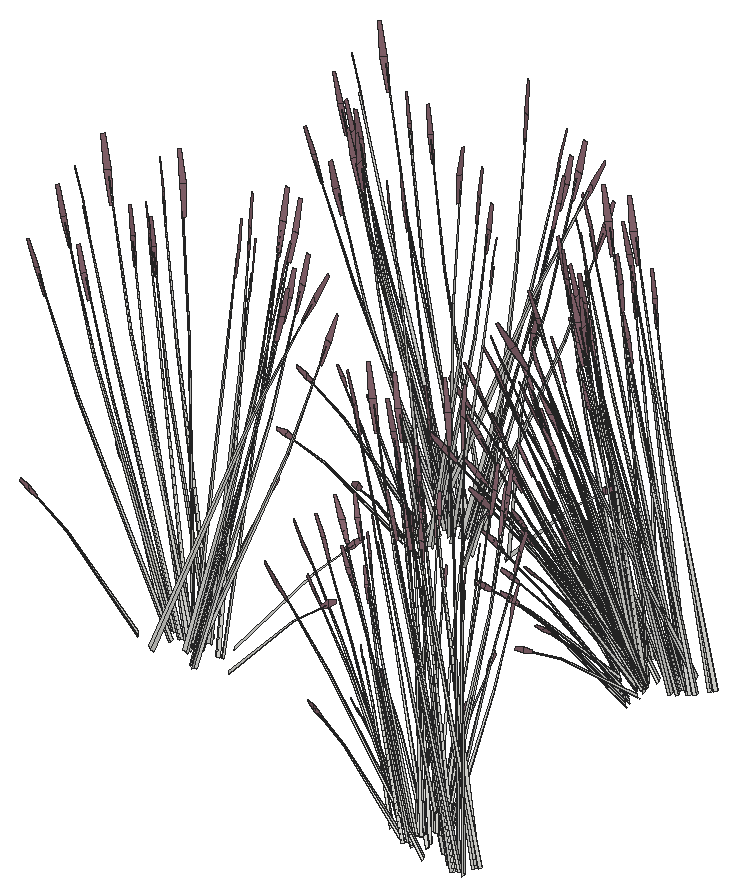
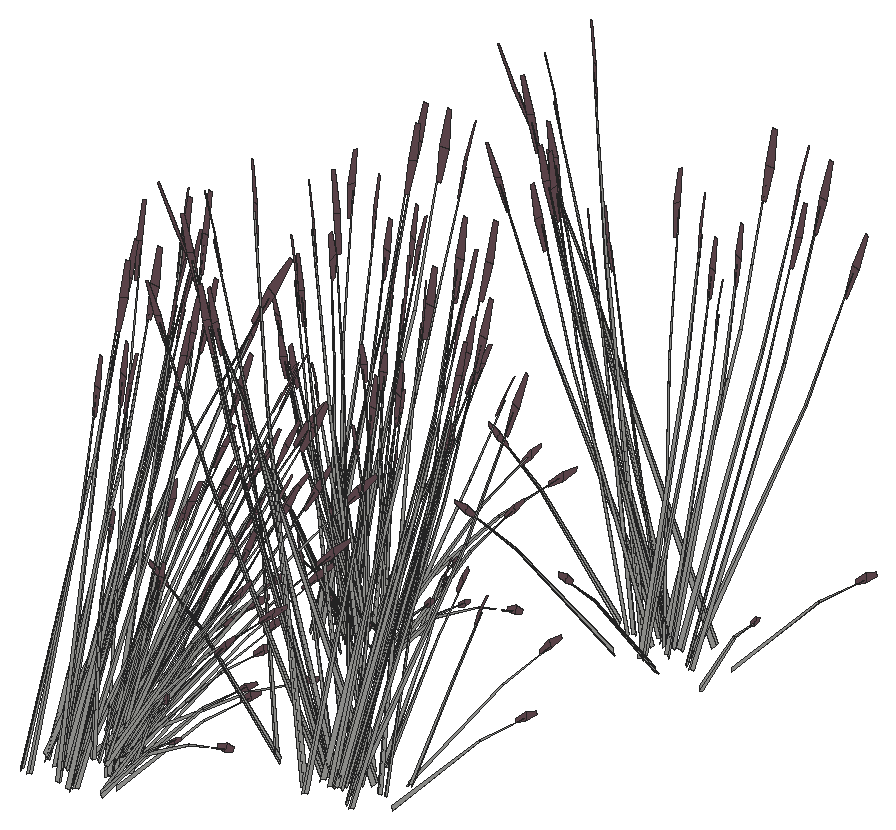
# SketchUp Ruby script. Lengths in inches.
U = 1.inch
M = Sketchup.active_model
def pt(a) = Geom::Point3d.new(a.map { |v| v * U })
def face(e, loops, mat)
  f = e.add_face(loops[0].map { |a| pt(a) })
  loops[1..].each { |l| e.add_face(l.map { |a| pt(a) }).erase! }
  f.material = f.back_material = mat if mat
  f
end
# faces: each face lists its corners as indices into pts; further lists are holes
def faces(e, pts, list, mat = nil) = list.each { |f| face(e, (f[0].is_a?(Array) ? f : [f]).map { |l| l.map { |i| pts[i] } }, mat) }
# xy, xz, yz: faces in a plane at the given z, y or x. An outline is a flat list of corners, or four numbers for a rectangle; further outlines are holes
def ring(l) = l.size == 4 ? [[l[0], l[1]], [l[2], l[1]], [l[2], l[3]], [l[0], l[3]]] : l.each_slice(2).to_a
def flat(e, list, mat, &to3) = list.each { |f| face(e, (f[0].is_a?(Array) ? f : [f]).map { |l| ring(l).map { |u, v| to3.(u, v) } }, mat) }
def xy(e, z, list, mat = nil) = flat(e, list, mat) { |x, y| [x, y, z] }
def xz(e, y, list, mat = nil) = flat(e, list, mat) { |x, z| [x, y, z] }
def yz(e, x, list, mat = nil) = flat(e, list, mat) { |y, z| [x, y, z] }
def lines(e, pts, list) = list.each { |a, b| e.add_line(pt(pts[a]), pt(pts[b])) }
# prism: a flat outline (further loops are holes) pulled along v
def prism(e, loops, v, mat = nil)
  f = face(e, loops, mat); d = Geom::Vector3d.new(v.map { |x| x * U })
  f.pushpull(f.normal.samedirection?(d) ? d.length : -d.length)
end
def box(e, o, s, mat = nil) = prism(e, [[o, [o[0] + s[0], o[1], o[2]], [o[0] + s[0], o[1] + s[1], o[2]], [o[0], o[1] + s[1], o[2]]]], [0, 0, s[2]], mat)
def at(x, y, z, deg = 0) = Geom::Transformation.translation(pt([x, y, z])) * Geom::Transformation.rotation(ORIGIN, Z_AXIS, deg.degrees)
def axes(o, x, y, z) = Geom::Transformation.new([*x, 0, *y, 0, *z, 0, *pt(o).to_a, 1])
def part(name) = M.definitions.add(name)
# library, detail: a bought-in or finely detailed component or shape, given as its bounding box
def library(name, o, s) = part(name).tap { |d| box(d.entities, o, s) }
def detail(e, o, s) = box(e.add_group.entities, o, s)
def put(e, d, t, mat = nil) = e.add_instance(d, t).tap { |i| i.material = mat if mat }
def group(e, t, mat = nil) = e.add_group.tap { |g| g.transformation = t; g.material = mat if mat }.entities
root = M.entities
M.materials.add("LightPink_Translucent").color = [144, 107, 117]
c1 = part("blade")
p = [[2.15,0.21,22],[0,0.17,0],[0.09,0.45,0],[2.18,0.31,22],[2.29,0.31,22],[0.38,0.45,0],
  [2.48,0.24,33],[2.49,0.24,33],[2.48,0.22,33]]
faces(c1.entities,p,[[0,1,2,3],[4,5,2,3],[6,3,4,7],[8,0,3,6]])
c2 = part("seeds")
p = [[0.3,-0.1,1.38],[-0.01,-0.03,1.59],[-0.01,-0.03,0.03],[0.14,-0.07,-0.07],[0.29,-0.03,3],[0.15,0.01,3.11]]
faces(c2.entities,p,[[0,1,2,3],[1,0,4,5]],"LightPink_Translucent")
c3 = part("blade with seeds")
put(c3.entities,c1,at(0,0,0))
put(c3.entities,c2,axes([2.4,0.25,30.99],[1.5799,-0.05474,1.17369],[-0.12525,1.92788,0.29478],[-0.07173,-0.02425,1.56792]))
put(root,c3,axes([28.59,392.67,43.49],[0.03108,0.16322,1.76342],[-0.62654,0.85237,-0.26939],[-0.44504,-0.04296,0.30037]))
put(root,c3,axes([28.26,397.24,43.49],[0.16438,0.10347,1.76342],[0.27873,0.95868,-0.26939],[-0.36432,0.20444,0.30037]))
put(root,c3,axes([32.69,394.15,44.06],[-1.27479,-0.1698,-0.62353],[0.26901,-1.04736,-0.16365],[-0.38043,-0.12691,1.37633]))
put(root,c3,axes([31.02,396.14,44.02],[-1.14694,-0.51783,-0.49651],[0.68554,-0.92854,0],[-0.26122,-0.11794,1.57504]))
put(root,c3,axes([34.14,394.31,44.67],[-1.23732,0.68758,-0.29095],[-0.8228,-0.97154,-0.50002],[-0.30528,-0.09867,1.59708]))
put(root,c3,axes([31.34,395.75,44.03],[-0.28787,-0.90242,-0.30978],[1.14332,-0.25625,0.30978],[-0.23049,-0.10406,1.38974]))
put(root,c3,axes([34.96,395.06,44.06],[-0.82544,0.77843,-0.62353],[-1.0254,-0.70586,-0.16365],[-0.33076,0.19418,1.37633]))
put(root,c3,axes([35.53,394.62,44.46],[-1.19666,-0.83357,-0.25192],[1.00694,-0.93603,0.5513],[-0.32224,0.09751,1.68216]))
put(root,c3,axes([36.74,432.36,43.49],[0.03108,0.16322,1.76342],[-0.62654,0.85237,-0.26939],[-0.44504,-0.04296,0.30037]))
put(root,c3,axes([34.92,394.44,44.21],[-1.33077,0.06393,-0.44739],[-0.12035,-1.06125,0.21531],[-0.23824,0.10756,1.43643]))
put(root,c3,axes([36.32,397.18,44.02],[-1.14694,0.51783,-0.49651],[-0.68554,-0.92854,0],[-0.26122,0.11794,1.57504]))
put(root,c3,axes([36.05,396.77,44.03],[-1.14332,-0.25625,-0.30978],[0.28787,-0.90242,0.30978],[-0.23049,0.10406,1.38974]))
put(root,c3,axes([35.85,394.16,44.67],[0.1428,1.18174,-0.29095],[-1.48733,0.07145,-0.50002],[-0.26191,0.15741,1.59708]))
put(root,c3,axes([40.84,433.84,44.06],[-1.27479,-0.1698,-0.62353],[0.26901,-1.04736,-0.16365],[-0.38043,-0.12691,1.37633]))
put(root,c3,axes([39.17,435.83,44.02],[-1.14694,-0.51783,-0.49651],[0.68554,-0.92854,0],[-0.26122,-0.11794,1.57504]))
put(root,c3,axes([38.67,428.11,43.49],[-0.11871,0.13643,1.76342],[-1.19964,0.29415,-0.26939],[-0.2898,-0.26759,0.30037]))
put(root,c3,axes([37.92,428.64,44.13],[-0.35352,0.84566,-0.03893],[-1.08806,-0.26014,-0.17649],[-0.1652,-0.13832,0.58215]))
put(root,c3,axes([33.33,397.34,43.49],[0.19833,-0.05635,1.76342],[1.19302,0.31018,-0.26939],[0.03489,0.3496,0.30037]))
put(root,c3,axes([42.29,434,44.67],[-1.23732,0.68758,-0.29095],[-0.8228,-0.97154,-0.50002],[-0.30528,-0.09867,1.59708]))
put(root,c3,axes([39.49,435.44,44.03],[-0.28787,-0.90242,-0.30978],[1.14332,-0.25625,0.30978],[-0.23049,-0.10406,1.38974]))
put(root,c3,axes([36.4,393.69,44.21],[-0.59459,0.93321,-0.44739],[-1.23546,-0.44912,0.21531],[0,0.21512,1.43643]))
put(root,c3,axes([43.68,434.3125,44.46],[-1.19666,-0.83357,-0.25192],[1.00694,-0.93603,0.5513],[-0.32224,0.09751,1.68216]))
put(root,c3,axes([41.5,433.51,44.21],[-0.73619,-0.86927,-0.44739],[1.11511,-0.61213,0.21531],[-0.23824,-0.10756,1.43643]))
put(root,c3,axes([43.07,434.14,44.21],[-1.33077,0.06393,-0.44739],[-0.12035,-1.06125,0.21531],[-0.23824,0.10756,1.43643]))
put(root,c3,axes([41.61,434.01,44.4375],[0.32481,-1.2272,-0.23429],[1.54007,0.21392,0.51271],[-0.26911,-0.16947,1.5644]))
put(root,c3,axes([37.68,431.71,44.02],[0,-1.03566,-0.49651],[1.37109,0,0],[0,-0.23588,1.57504]))
put(root,c3,axes([39.54,394.09,44.03],[-0.85545,0.64616,-0.30978],[-0.85545,-0.64616,0.30978],[0,0.20813,1.38974]))
put(root,c3,axes([37.09,393.98,44.09],[0.44936,0.94823,-0.69212],[-1.29441,0.3415,-0.18165],[0.04967,0.32109,1.52773]))
put(root,c3,axes([44.2,436.46,44.03],[-1.14332,-0.25625,-0.30978],[0.28787,-0.90242,0.30978],[-0.23049,0.10406,1.38974]))
put(root,c3,axes([41.26,432.91,44.67],[-1.38012,-0.49416,-0.29095],[0.66454,-1.04299,-0.50002],[-0.04337,-0.25608,1.59708]))
put(root,c3,axes([36.54,392.92,44.67],[1.38012,0.49416,-0.29095],[-0.66454,1.04299,-0.50002],[0.04337,0.25608,1.59708]))
put(root,c3,axes([40.65,431.86,44.1],[-0.50328,-1.06202,-0.69835],[1.44974,-0.38248,-0.18329],[-0.05563,-0.35963,1.54149]))
put(root,c3,axes([38.27,431.74,44.03],[0.85545,-0.64616,-0.30978],[0.85545,0.64616,0.30978],[0,-0.20813,1.38974]))
put(root,c3,axes([42.13,427.56,44.13],[-0.84686,0.59414,-0.03893],[-0.77596,-0.65071,-0.17649],[-0.05463,-0.18438,0.58215]))
put(root,c3,axes([40.125,394.12,44.02],[0,1.03566,-0.49651],[-1.37109,0,0],[0,0.23588,1.57504]))
put(root,c3,axes([36.28,395.33,44.18],[1.2866,-0.3514,-0.19198],[0.45209,1.01223,0.00008],[0.14202,-0.03884,1.73897]))
put(root,c3,axes([36.3,392.32,44.21],[0.73619,0.86927,-0.44739],[-1.11511,0.61213,0.21531],[0.23824,0.10756,1.43643]))
put(root,c3,axes([42.34,426.83,43.49],[-0.20555,0.03731,1.76342],[-1.13672,-0.42002,-0.26939],[0.01907,-0.35034,0.30037]))
put(root,c3,axes([41.41,432.14,44.21],[0.59459,-0.93321,-0.44739],[1.23546,0.44912,0.21531],[0,-0.21512,1.43643]))
put(root,c3,axes([38.32,390.39,44.03],[0.28787,0.90242,-0.30978],[-1.14332,0.25625,0.30978],[0.23049,0.10406,1.38974]))
put(root,c3,axes([35.52,391.83,44.67],[1.23732,-0.68758,-0.29095],[0.8228,0.97154,-0.50002],[0.30528,0.09867,1.59708]))
put(root,c3,axes([32.39,391.22,43.59],[-1.20625,0.41464,1.28929],[-0.38394,-1.1897,0.50096],[0.74071,0.01979,1.46642]))
put(root,c3,axes([38.64,390,44.02],[1.14694,0.51783,-0.49651],[-0.68554,0.92854,0],[0.26122,0.11794,1.57504]))
put(root,c3,axes([38.58,397.37,43.49],[0.08928,-0.14952,1.76342],[1.12407,-0.44035,-0.26939],[0.34078,0.22791,0.30037]))
put(root,c3,axes([36.96,391.99,44.06],[1.27479,0.1698,-0.62353],[-0.26901,1.04736,-0.16365],[0.38043,0.12691,1.37633]))
put(root,c3,axes([41.95,431.67,44.67],[-0.1428,-1.18174,-0.29095],[1.48733,-0.07145,-0.50002],[0.26191,-0.15741,1.59708]))
put(root,c3,axes([41.76,429.06,44.03],[1.14332,0.25625,-0.30978],[-0.28787,0.90242,0.30978],[0.23049,-0.10406,1.38974]))
put(root,c3,axes([41.49,428.65,44.02],[1.14694,-0.51783,-0.49651],[0.68554,0.92854,0],[0.26122,-0.11794,1.57504]))
put(root,c3,axes([44.43,435.02,44.18],[1.2866,-0.3514,-0.19198],[0.45209,1.01223,0.00008],[0.14202,-0.03884,1.73897]))
put(root,c3,axes([44.46,432.01,44.21],[0.73619,0.86927,-0.44739],[-1.11511,0.61213,0.21531],[0.23824,0.10756,1.43643]))
put(root,c3,axes([41.82,392.83,43.49],[-0.06405,-0.15723,1.76342],[0.44421,-0.91974,-0.26939],[0.4481,-0.01323,0.30037]))
put(root,c3,axes([42.85,430.77,44.06],[0.82544,-0.77843,-0.62353],[1.0254,0.70586,-0.16365],[0.33076,-0.19418,1.37633]))
put(root,c3,axes([46.47,430.08,44.03],[0.28787,0.90242,-0.30978],[-1.14332,0.25625,0.30978],[0.23049,0.10406,1.38974]))
put(root,c3,axes([43.67,431.52,44.67],[1.23732,-0.68758,-0.29095],[0.8228,0.97154,-0.50002],[0.30528,0.09867,1.59708]))
put(root,c3,axes([40.55,430.91,43.59],[-1.20625,0.41464,1.28929],[-0.38394,-1.1897,0.50096],[0.74071,0.01979,1.46642]))
put(root,c3,axes([47.375,428.62,43.49],[-0.18342,-0.08159,1.76342],[-0.47115,-0.9115,-0.26939],[0.31784,-0.24736,0.30037]))
put(root,c3,axes([46.79,429.7,44.02],[1.14694,0.51783,-0.49651],[-0.68554,0.92854,0],[0.26122,0.11794,1.57504]))
put(root,c3,axes([45.12,431.68,44.06],[1.27479,0.1698,-0.62353],[-0.26901,1.04736,-0.16365],[0.38043,0.12691,1.37633]))
put(root,c3,axes([50.54,432.3,44.26],[-0.75977,-0.66224,-0.06488],[0.83212,-0.6068,-0.29416],[0.23578,-0.04272,0.97024]))
put(root,c3,axes([69.75,430.67,36.3],[0.50831,-0.02346,1.71376],[-0.33721,1.01661,0.13857],[-0.72439,-0.06288,0.73262]))
put(root,c3,axes([49.97,432.53,43.49],[-0.06405,-0.15723,1.76342],[0.44421,-0.91974,-0.26939],[0.4481,-0.01323,0.30037]))
put(root,c3,axes([69.96,389.98,32.11],[0.42521,-0.21906,1.71376],[0.35798,1.01226,0.13857],[-0.66754,0.22878,0.73262]))
put(root,c3,axes([69.96,432.46,36.3],[0.42521,-0.21906,1.71376],[0.35798,1.01226,0.13857],[-0.66754,0.22878,0.73262]))
put(root,c3,axes([68.64,391.7,30.83],[0.42589,0.08502,1.43002],[0.2745,0.86839,-0.30754],[-0.57851,0.16255,0.61141]))
put(root,c3,axes([68.64,434.1875,35.02],[0.42589,0.08502,1.43002],[0.2745,0.86839,-0.30754],[-0.57851,0.16255,0.61141]))
put(root,c3,axes([72.41,388.92,31.58],[0.34834,-0.14982,1.77064],[0.12012,1.04605,0.13857],[-0.75452,0.1388,0.63284]))
put(root,c3,axes([72.41,431.41,35.77],[0.34834,-0.14982,1.77064],[0.12012,1.04605,0.13857],[-0.75452,0.1388,0.63284]))
put(root,c3,axes([68.66,389.62,32.95],[-0.20012,0.13446,1.74944],[0.01702,0.98243,-0.27667],[-0.45871,0.12776,0.14031]))
put(root,c3,axes([68.66,432.11,37.14],[-0.20012,0.13446,1.74944],[0.01702,0.98243,-0.27667],[-0.45871,0.12776,0.14031]))
put(root,c3,axes([71.27,429.73,37.41],[-1.22504,-0.02494,-0.71045],[0.08228,-1.05005,0.08574],[-0.51899,-0.11081,1.00501]))
put(root,c3,axes([70.29,429.98,35.02],[0.23927,0.28834,1.43002],[-0.55135,0.78376,-0.30754],[-0.56612,-0.18733,0.61141]))
put(root,c3,axes([69.31,431.55,36.95],[-1.01846,-0.28891,-0.35414],[0.29705,-0.84289,0.4572],[-0.41005,0.07729,0.87481]))
put(root,c3,axes([70.71,429.04,36.3],[0.45521,0.17844,1.71376],[-0.94204,0.74856,0.13857],[-0.58713,-0.33769,0.73262]))
put(root,c3,axes([66.4375,390.62,32.95],[0.1564,0.02778,1.77383],[0.48382,0.91506,-0.16761],[-0.32016,0.24017,0.31391]))
put(root,c3,axes([66.4375,433.1,37.14],[0.1564,0.02778,1.77383],[0.48382,0.91506,-0.16761],[-0.32016,0.24017,0.31391]))
put(root,c3,axes([70,389.49,32.92],[-0.332,0.94205,-0.51099],[-1.13828,-0.3229,-0.3958],[-0.45829,0.08638,0.97773]))
put(root,c3,axes([70,431.98,37.11],[-0.332,0.94205,-0.51099],[-1.13828,-0.3229,-0.3958],[-0.45829,0.08638,0.97773]))
put(root,c3,axes([70.87,429.94,37.11],[-0.88986,0.68603,-0.51099],[-0.77932,-0.72471,-0.3958],[-0.45212,-0.10438,0.97773]))
put(root,c3,axes([69.43,431.92,33.92],[0.03108,0.16322,1.76342],[-0.62654,0.85237,-0.26939],[-0.44504,-0.04296,0.30037]))
put(root,c3,axes([69.61,428.02,37.14],[0.09085,0.10335,1.77383],[-0.43798,0.92907,-0.16761],[-0.44357,0.00672,0.31391]))
put(root,c3,axes([67.75,393.52,31],[0.51072,-0.46938,1.1486],[0.20153,0.74307,0.84392],[-0.36908,0.13305,0.25299]))
put(root,c3,axes([67.75,436.01,35.19],[0.51072,-0.46938,1.1486],[0.20153,0.74307,0.84392],[-0.36908,0.13305,0.25299]))
put(root,c3,axes([70.625,427.4,37.14],[-0.26368,-0.00731,1.74944],[-0.83946,0.73103,-0.27667],[-0.44791,-0.14937,0.14031]))
put(root,c3,axes([69.54,431.44,37.16],[0.34623,-0.9443,0.48003],[1.13828,0.3229,0.3958],[-0.44763,0.05675,0.9933]))
put(root,c3,axes([69.95,388.6875,33.27],[0.6166,0.93779,-0.1216],[-1.09436,0.46085,-0.67495],[-0.46117,0.12373,1.02557]))
put(root,c3,axes([69.95,431.17,37.46],[0.6166,0.93779,-0.1216],[-1.09436,0.46085,-0.67495],[-0.46117,0.12373,1.02557]))
put(root,c3,axes([71.33,429.22,37.46],[-0.06562,1.05324,-0.1216],[-1.2424,-0.02879,-0.67495],[-0.4785,-0.07316,1.02557]))
put(root,c3,axes([70.54,429.3,36.95],[-0.69728,-0.64842,-0.35414],[0.79619,-0.61382,0.4572],[-0.40453,-0.09339,0.87481]))
put(root,c3,axes([69.46,431.19,37.16],[-0.4501,-0.70615,0.0643],[0.82077,-0.34564,0.50621],[-0.36181,0.0682,0.77189]))
put(root,c3,axes([71.52,390.66,32.11],[0.30609,-0.31822,1.71376],[0.77286,0.85893,0.13857],[-0.53009,0.39116,0.73262]))
put(root,c3,axes([69.68,391.49,32.76],[-1.06674,0.14801,-0.35414],[-0.28168,-0.84611,0.4572],[-0.30569,0.22726,0.87481]))
put(root,c3,axes([69.1,394,29.73],[0.16438,0.10347,1.76342],[0.27873,0.95868,-0.26939],[-0.36432,0.20444,0.30037]))
put(root,c3,axes([68.86,430.85,35.19],[0.78239,-0.07411,1.1486],[-0.49629,0.65296,0.84392],[-0.38663,-0.09795,0.25299]))
put(root,c3,axes([69.82,391.31,32.97],[-0.30393,-0.95317,0.48003],[1.19224,-0.16542,0.3958],[-0.35138,0.22417,0.9933]))
put(root,c3,axes([69.82,433.79,37.16],[-0.30393,-0.95317,0.48003],[1.19224,-0.16542,0.3958],[-0.35138,0.22417,0.9933]))
put(root,c3,axes([70.43,429.05,37.52],[1.01205,-0.7643,0.53763],[0.87284,0.81167,0.4433],[-0.47482,-0.14098,1.11249]))
put(root,c3,axes([69.58,391.125,32.97],[-0.8413,-0.43556,0.0643],[0.48981,-0.62025,0.50621],[-0.26973,0.20053,0.77189]))
put(root,c3,axes([69.58,433.61,37.16],[-0.8413,-0.43556,0.0643],[0.48981,-0.62025,0.50621],[-0.26973,0.20053,0.77189]))
put(root,c3,axes([71.29,391.44,32.11],[0.22818,-0.35597,1.71376],[0.95725,0.73667,0.13857],[-0.43183,0.45914,0.73262]))
put(root,c3,axes([70.38,388.97,33.29],[1.01846,0.28891,0.35414],[-0.29705,0.84289,-0.4572],[-0.41005,0.07729,0.87481]))
put(root,c3,axes([70.38,431.45,37.48],[1.01846,0.28891,0.35414],[-0.29705,0.84289,-0.4572],[-0.41005,0.07729,0.87481]))
put(root,c3,axes([70.56,391.59,32.92],[0.31482,0.94565,-0.51099],[-1.19224,0.16542,-0.3958],[-0.34166,0.254,0.97773]))
put(root,c3,axes([70.89,429.05,37.16],[0.06171,-0.78753,0.0643],[0.9318,0.02159,0.50621],[-0.35694,-0.08241,0.77189]))
put(root,c3,axes([68.7,393.29,32.95],[-0.03046,0.20495,1.74944],[0.86449,0.71297,-0.27667],[-0.22632,0.33716,0.14031]))
put(root,c3,axes([73.53,433.4,34.49],[-1.27479,-0.1698,-0.62353],[0.26901,-1.04736,-0.16365],[-0.38043,-0.12691,1.37633]))
put(root,c3,axes([73.76,427.68,37.86],[-0.81789,0.99285,-0.13619],[-1.18445,-0.572,-0.75594],[-0.41173,-0.28051,1.14864]))
put(root,c3,axes([71.53,429.63,37.48],[0.69728,0.64842,0.35414],[-0.79619,0.61382,-0.4572],[-0.40453,-0.09339,0.87481]))
put(root,c3,axes([73.4,428.49,37.41],[-1.04497,-0.50058,-0.71045],[0.74264,-0.8772,0.08574],[-0.3786,-0.29889,1.00501]))
put(root,c3,axes([72.91,428.52,37.11],[-1.20928,0.24619,-0.51099],[-0.21154,-0.93233,-0.3958],[-0.32481,-0.26718,0.97773]))
put(root,c3,axes([71.86,435.38,34.45],[-1.14694,-0.51783,-0.49651],[0.68554,-0.92854,0],[-0.26122,-0.11794,1.57504]))
put(root,c3,axes([71.35,427.67,33.92],[-0.11871,0.13643,1.76342],[-1.19964,0.29415,-0.26939],[-0.2898,-0.26759,0.30037]))
put(root,c3,axes([70,390.91,33.27],[1.1336,0.57106,-0.1216],[-0.65308,0.827,-0.67495],[-0.32027,0.28747,1.02557]))
put(root,c3,axes([72.56,393.52,30.61],[-0.7662,1.03778,0],[-1.28187,-0.57875,-0.51607],[-0.29196,-0.13181,1.63711]))
put(root,c3,axes([72.56,436,34.8],[-0.7662,1.03778,0],[-1.28187,-0.57875,-0.51607],[-0.29196,-0.13181,1.63711]))
put(root,c3,axes([68.125,393.39,33.88],[1.08141,0.27645,-0.06488],[-0.33265,0.85086,-0.29416],[-0.17688,0.12919,0.97024]))
put(root,c3,axes([70.55,390.99,33.29],[1.06674,-0.14801,0.35414],[0.28168,0.84611,-0.4572],[-0.30569,0.22726,0.87481]))
put(root,c3,axes([70.55,433.48,37.48],[1.06674,-0.14801,0.35414],[0.28168,0.84611,-0.4572],[-0.30569,0.22726,0.87481]))
put(root,c3,axes([71.16,395.02,30.83],[0.38672,-0.16338,1.43002],[0.95481,0.49262,-0.30754],[-0.28419,0.42626,0.61141]))
put(root,c3,axes([70.61,428.19,34.56],[-0.35352,0.84566,-0.03893],[-1.08806,-0.26014,-0.17649],[-0.1652,-0.13832,0.58215]))
put(root,c3,axes([73.44,425.32,37.14],[-0.02286,0.12414,1.77383],[-1.12758,0.45052,-0.16761],[-0.33182,-0.23029,0.31391]))
put(root,c3,axes([72.23,427.125,35.02],[-0.07421,0.33879,1.43002],[-1.08488,0.28361,-0.30754],[-0.25359,-0.4379,0.61141]))
put(root,c3,axes([72.59,428,36.3],[0.28013,0.33252,1.71376],[-1.29445,0.27994,0.13857],[-0.29256,-0.52202,0.73262]))
put(root,c3,axes([74.98,433.55,35.09],[-1.23732,0.68758,-0.29095],[-0.8228,-0.97154,-0.50002],[-0.30528,-0.09867,1.59708]))
put(root,c3,axes([71.56,393.24,32.97],[-0.87265,-0.70663,0.48003],[0.92674,-0.60943,0.3958],[-0.16097,0.33153,0.9933]))
put(root,c3,axes([73.04,427.83,36.95],[-0.18927,-0.83419,-0.35414],[1.08199,-0.22027,0.4572],[-0.29062,-0.23905,0.87481]))
put(root,c3,axes([70.02,432.05,34.8],[-1.53239,0,0],[0,-1.1575,-0.51607],[0,-0.26363,1.63711]))
put(root,c3,axes([72.18,434.99,34.46],[-0.28787,-0.90242,-0.30978],[1.14332,-0.25625,0.30978],[-0.23049,-0.10406,1.38974]))
put(root,c3,axes([71.24,393.17,32.97],[-1.00708,-0.04826,0.0643],[0.02761,-0.72867,0.50621],[-0.10538,0.27912,0.77189]))
put(root,c3,axes([71.55,393.45,32.76],[-0.82919,0.54528,-0.35414],[-0.78493,-0.62262,0.4572],[-0.11943,0.31634,0.87481]))
put(root,c3,axes([75.8,391.82,30.3],[-0.82544,0.77843,-0.62353],[-1.0254,-0.70586,-0.16365],[-0.33076,0.19418,1.37633]))
put(root,c3,axes([73.68,428.51,37.48],[0.18927,0.83419,0.35414],[-1.08199,0.22027,-0.4572],[-0.29062,-0.23905,0.87481]))
put(root,c3,axes([68.6,395.39,32.95],[0.13903,-0.06253,1.77383],[1.14912,0.41591,-0.16761],[-0.027,0.34629,0.31391]))
put(root,c3,axes([71.21,431.75,34.76],[-1.1399,0.87071,0.30756],[-1.1406,-0.86155,-0.36492],[-0.03981,-0.24727,1.64885]))
put(root,c3,axes([75.9,434.15,35.75],[1.05902,0.41762,1.51261],[-1.03748,0.89969,0.59816],[-0.46471,-0.53324,1.26806]))
put(root,c3,axes([71.86,426.58,35.19],[0.63926,0.36046,1.1486],[-0.93099,0.21668,0.84392],[-0.1992,-0.27702,0.25299]))
put(root,c3,axes([76.37,391.38,30.7],[-1.19666,-0.83357,-0.25192],[1.00694,-0.93603,0.5513],[-0.32224,0.09751,1.68216]))
put(root,c3,axes([76.37,433.87,34.89],[-1.19666,-0.83357,-0.25192],[1.00694,-0.93603,0.5513],[-0.32224,0.09751,1.68216]))
put(root,c3,axes([74.19,433.0625,34.64],[-0.73619,-0.86927,-0.44739],[1.11511,-0.61213,0.21531],[-0.23824,-0.10756,1.43643]))
put(root,c3,axes([72.11,392.875,33.57],[-0.03189,0.95798,-0.7886],[-1.34277,-0.06434,0.09517],[-0.14171,0.40585,1.11556]))
put(root,c3,axes([72.08,395.57,31],[-0.03171,-0.6158,1.1486],[0.7925,0.43922,0.84392],[-0.15586,0.29352,0.25299]))
put(root,c3,axes([73.2,427.53,37.52],[1.36515,-0.26619,0.53763],[0.23692,1.04421,0.4433],[-0.32106,-0.30775,1.11249]))
put(root,c3,axes([75.76,391.2,30.45],[-1.33077,0.06393,-0.44739],[-0.12035,-1.06125,0.21531],[-0.23824,0.10756,1.43643]))
put(root,c3,axes([75.76,433.6875,34.64],[-1.33077,0.06393,-0.44739],[-0.12035,-1.06125,0.21531],[-0.23824,0.10756,1.43643]))
put(root,c3,axes([73.51,427.75,37.16],[0.55698,-0.6579,0.0643],[0.79316,0.38303,0.50621],[-0.25643,-0.21093,0.77189]))
put(root,c3,axes([73.22,392.98,30.71],[1.14694,0.51783,0.49651],[-0.68554,0.92854,0],[-0.26122,-0.11794,1.57504]))
put(root,c3,axes([73.22,435.46,34.91],[1.14694,0.51783,0.49651],[-0.68554,0.92854,0],[-0.26122,-0.11794,1.57504]))
put(root,c3,axes([71.66,394.22,31.6],[0.02693,-0.53464,1.54345],[1.21102,0.2824,0.21329],[-0.10493,0.5698,0.72882]))
put(root,c3,axes([74.3,433.5625,34.87],[0.32481,-1.2272,-0.23429],[1.54007,0.21392,0.51271],[-0.26911,-0.16947,1.5644]))
put(root,c3,axes([74.86,391.37,30.85],[-0.23642,0.92427,0.1448],[-1.15506,-0.16044,-0.41347],[-0.21021,-0.09491,1.26744]))
put(root,c3,axes([74.86,433.85,35.04],[-0.23642,0.92427,0.1448],[-1.15506,-0.16044,-0.41347],[-0.21021,-0.09491,1.26744]))
put(root,c3,axes([74.73,425.8,37.14],[-0.18744,-0.14521,1.74944],[-1.25089,0.09206,-0.27667],[-0.19964,-0.34731,0.14031]))
put(root,c3,axes([77.16,393.94,30.25],[-1.14694,0.51783,-0.49651],[-0.68554,-0.92854,0],[-0.26122,0.11794,1.57504]))
put(root,c3,axes([70.37,431.27,34.45],[0,-1.03566,-0.49651],[1.37109,0,0],[0,-0.23588,1.57504]))
put(root,c3,axes([70.95,432.23,34.91],[0,1.03566,0.49651],[-1.37109,0,0],[0,-0.23588,1.57504]))
put(root,c3,axes([77.23,393.66,30.43],[-0.75665,-1.04141,-0.05142],[1.28187,-0.57875,0.51607],[-0.31588,0.09915,1.6363]))
put(root,c3,axes([77.23,436.15,34.62],[-0.75665,-1.04141,-0.05142],[1.28187,-0.57875,0.51607],[-0.31588,0.09915,1.6363]))
put(root,c3,axes([72.38,393.19,33.24],[0.87728,0.69587,-0.5672],[-0.92674,0.60943,-0.43934],[-0.13348,0.35356,1.08528]))
put(root,c3,axes([76.89,393.53,30.26],[-1.14332,-0.25625,-0.30978],[0.28787,-0.90242,0.30978],[-0.23049,0.10406,1.38974]))
put(root,c3,axes([76.89,436.02,34.46],[-1.14332,-0.25625,-0.30978],[0.28787,-0.90242,0.30978],[-0.23049,0.10406,1.38974]))
put(root,c3,axes([71.99,392.68,33.29],[0.82919,-0.54528,0.35414],[0.78493,0.62262,-0.4572],[-0.11943,0.31634,0.87481]))
put(root,c3,axes([73.95,432.47,35.09],[-1.38012,-0.49416,-0.29095],[0.66454,-1.04299,-0.50002],[-0.04337,-0.25608,1.59708]))
put(root,c3,axes([77.55,389.67,31.08],[-0.03348,-0.97511,1.41272],[1.51511,0.25277,0.59816],[-0.35835,0.53357,1.3335]))
put(root,c3,axes([71.46,392.83,33.63],[1.34686,0.05131,-0.13498],[-0.03681,0.97156,-0.74919],[-0.09356,0.37418,1.13838]))
put(root,c3,axes([71.43,394.24,31.06],[1.11329,-0.1834,0.06507],[0.25594,0.73887,-0.86304],[-0.07058,0.37403,0.7736]))
put(root,c3,axes([76.69,390.92,30.9],[0.1428,1.18174,-0.29095],[-1.48733,0.07145,-0.50002],[-0.26191,0.15741,1.59708]))
